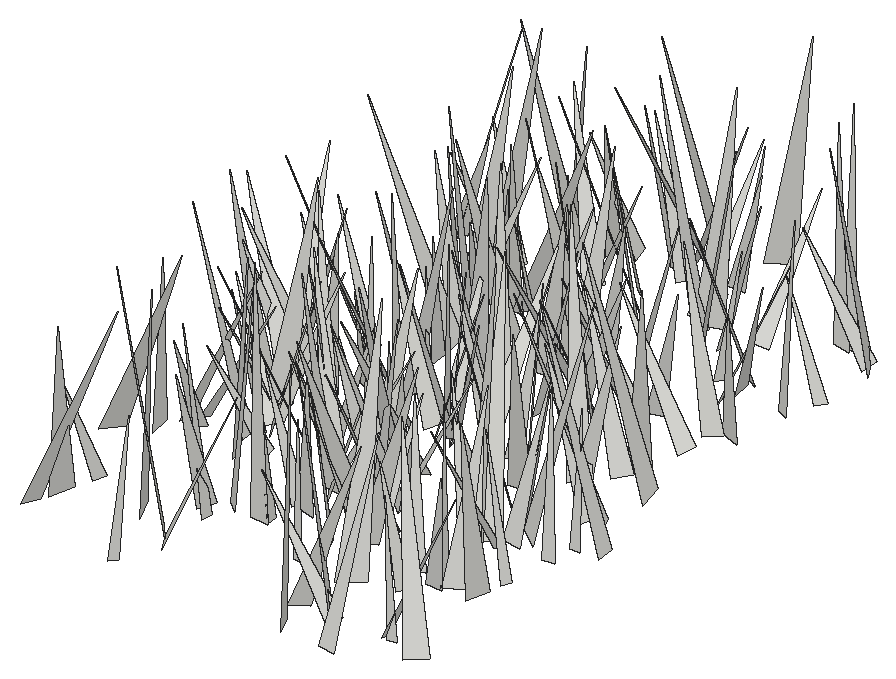
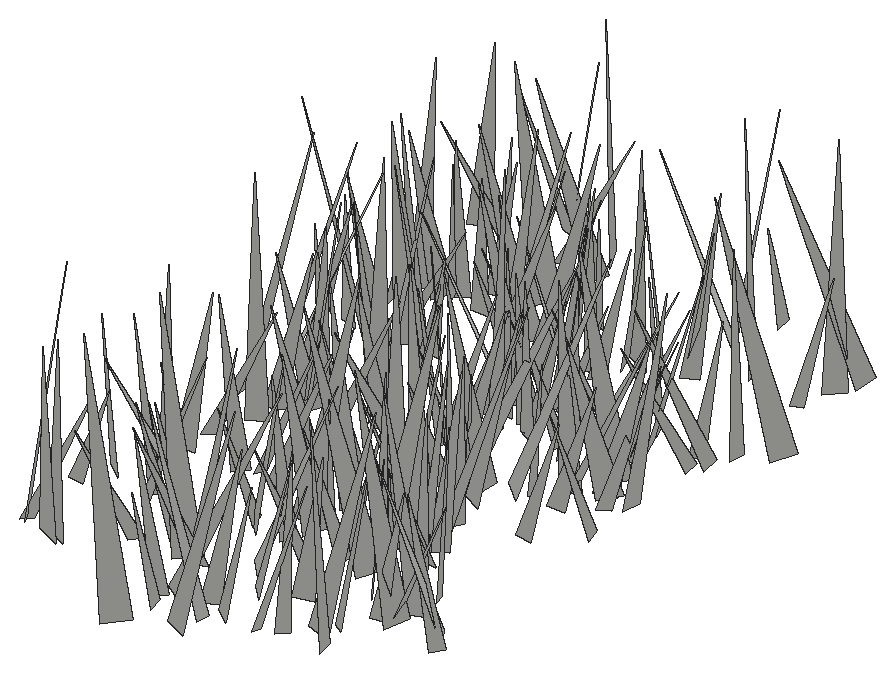
# SketchUp Ruby script. Lengths in inches.
U = 1.inch
M = Sketchup.active_model
def pt(a) = Geom::Point3d.new(a.map { |v| v * U })
def face(e, loops, mat)
  f = e.add_face(loops[0].map { |a| pt(a) })
  loops[1..].each { |l| e.add_face(l.map { |a| pt(a) }).erase! }
  f.material = f.back_material = mat if mat
  f
end
# faces: each face lists its corners as indices into pts; further lists are holes
def faces(e, pts, list, mat = nil) = list.each { |f| face(e, (f[0].is_a?(Array) ? f : [f]).map { |l| l.map { |i| pts[i] } }, mat) }
# xy, xz, yz: faces in a plane at the given z, y or x. An outline is a flat list of corners, or four numbers for a rectangle; further outlines are holes
def ring(l) = l.size == 4 ? [[l[0], l[1]], [l[2], l[1]], [l[2], l[3]], [l[0], l[3]]] : l.each_slice(2).to_a
def flat(e, list, mat, &to3) = list.each { |f| face(e, (f[0].is_a?(Array) ? f : [f]).map { |l| ring(l).map { |u, v| to3.(u, v) } }, mat) }
def xy(e, z, list, mat = nil) = flat(e, list, mat) { |x, y| [x, y, z] }
def xz(e, y, list, mat = nil) = flat(e, list, mat) { |x, z| [x, y, z] }
def yz(e, x, list, mat = nil) = flat(e, list, mat) { |y, z| [x, y, z] }
def lines(e, pts, list) = list.each { |a, b| e.add_line(pt(pts[a]), pt(pts[b])) }
# prism: a flat outline (further loops are holes) pulled along v
def prism(e, loops, v, mat = nil)
  f = face(e, loops, mat); d = Geom::Vector3d.new(v.map { |x| x * U })
  f.pushpull(f.normal.samedirection?(d) ? d.length : -d.length)
end
def box(e, o, s, mat = nil) = prism(e, [[o, [o[0] + s[0], o[1], o[2]], [o[0] + s[0], o[1] + s[1], o[2]], [o[0], o[1] + s[1], o[2]]]], [0, 0, s[2]], mat)
def at(x, y, z, deg = 0) = Geom::Transformation.translation(pt([x, y, z])) * Geom::Transformation.rotation(ORIGIN, Z_AXIS, deg.degrees)
def axes(o, x, y, z) = Geom::Transformation.new([*x, 0, *y, 0, *z, 0, *pt(o).to_a, 1])
def part(name) = M.definitions.add(name)
# library, detail: a bought-in or finely detailed component or shape, given as its bounding box
def library(name, o, s) = part(name).tap { |d| box(d.entities, o, s) }
def detail(e, o, s) = box(e.add_group.entities, o, s)
def put(e, d, t, mat = nil) = e.add_instance(d, t).tap { |i| i.material = mat if mat }
def group(e, t, mat = nil) = e.add_group.tap { |g| g.transformation = t; g.material = mat if mat }.entities
root = M.entities
c1 = part("fur_instance\#9")
p = [[0.8125,0,1.79],[0.67,-0.02,1.48],[0,-0.11,0],[0,0.11,0]]
faces(c1.entities,p,[[0,1,2,3]])
put(root,c1,axes([478.71,327.85,-21.66],[-6.33484,-0.15602,2.15214],[0.09289,6.64883,0.75543],[2.15578,-0.74496,6.29157]))
put(root,c1,axes([477.64,320.11,-21.66],[5.74214,0.07937,1.80023],[0.34922,-5.94743,-0.85168],[-1.76782,-0.91707,5.67918]))
put(root,c1,axes([478.67,313.66,-21.66],[2.63547,-2.52355,0.88422],[-2.24578,-2.7628,-1.19134],[-1.45143,-0.30736,3.44888]))
put(root,c1,axes([477.66,345.35,-21.66],[5.27233,3.79468,0.9806],[3.62511,-5.34626,1.19781],[-1.48988,0.42019,6.38454]))
put(root,c1,axes([480.66,327.67,-21.66],[-3.78677,4.88862,0.77178],[4.90876,3.58599,1.37062],[-0.63111,-1.44081,6.0299]))
put(root,c1,axes([477.02,346.69,-21.66],[2.31724,-3.70248,0.25487],[-3.62607,-2.19471,1.08527],[0.79054,0.78602,4.23086]))
put(root,c1,axes([475.72,318.5,-21.66],[6.5822,-3.48627,0.04021],[-3.46978,-6.5418,0.80411],[0.34104,0.72931,7.40492]))
put(root,c1,axes([479.73,328.98,-21.66],[-4.18916,1.41328,1.44955],[1.84035,4.04661,1.3732],[0.84361,-1.80976,4.20247]))
put(root,c1,axes([478.39,331.58,-21.66],[4.03699,1.00135,1.00845],[0.75439,-4.0837,1.03503],[-1.2044,0.79854,4.02849]))
put(root,c1,axes([477.99,311.26,-21.66],[6.15158,-3.29467,0.71793],[-3.15743,-6.15236,-1.17953],[-1.18361,-0.7112,6.87789]))
put(root,c1,axes([480.25,327.79,-21.66],[-4.33285,5.33033,0.39838],[5.19442,4.31986,-1.30443],[1.26061,0.52067,6.74422]))
put(root,c1,axes([479.34,321.4375,-21.66],[2.09335,-3.21544,0.11512],[-3.16402,-2.08217,-0.6229],[-0.58423,-0.24481,3.78592]))
put(root,c1,axes([481.14,334.13,-21.66],[-1.35537,3.98703,1.26023],[4.07237,0.95801,1.34893],[-0.94888,-1.58348,3.98921]))
put(root,c1,axes([477.34,309.4,-21.66],[6.84085,-1.05323,0.60817],[-1.14548,-6.7472,1.19982],[-0.40871,1.28156,6.81667]))
put(root,c1,axes([481.98,322.28,-21.66],[-6.45817,-1.9042,0.82118],[-2.02073,6.38203,-1.093],[0.4658,1.28531,6.64374]))
put(root,c1,axes([480.9,345.43,-21.66],[-3.67924,-0.76157,0.35539],[-0.68587,3.64327,0.70657],[0.48566,-0.62424,3.6902]))
put(root,c1,axes([478.27,321.625,-21.66],[5.14686,-0.10254,0.48257],[-0.21946,-5.00543,1.27711],[-0.44184,1.29176,4.98695]))
put(root,c1,axes([482.23,328.67,-21.66],[-5.87087,-0.65311,0.1721],[-0.62527,5.82501,0.77566],[0.25536,-0.75237,5.85594]))
put(root,c1,axes([481.77,330.56,-21.66],[-2.38269,3.95567,1.05235],[4.03891,2.07425,1.34786],[-0.66484,-1.57548,4.41677]))
put(root,c1,axes([482.22,324.16,-21.66],[-3.14834,2.92622,0.07201],[2.87738,3.07451,0.86494],[-0.53726,-0.68166,4.21031]))
put(root,c1,axes([478.875,322.49,-21.66],[4.0967,-0.1052,0.02727],[-0.10864,-3.93802,1.12914],[0.00278,1.12946,3.93942]))
put(root,c1,axes([481.6,346,-21.66],[1.42744,-3.53628,2.17287],[-3.81125,-2.02664,-0.79456],[-1.64348,1.62839,3.72982]))
put(root,c1,axes([480.47,342.17,-21.66],[4.23333,1.58778,2.03705],[2.11026,-4.38143,-0.97034],[-1.48911,-1.69519,4.41595]))
put(root,c1,axes([482.51,322.92,-21.66],[-3.84784,-1.19504,0.32807],[-1.23606,3.62421,-1.29571],[-0.08892,1.33363,3.81512]))
put(root,c1,axes([481.8,325.32,-21.66],[-3.17916,-2.57933,0.00353],[-2.53731,3.12837,0.73174],[0.46373,-0.56605,4.02798]))
put(root,c1,axes([480.21,344.3,-21.66],[0.14436,6.2225,2.72909],[6.68972,0.34776,-1.14678],[1.18962,-2.71069,6.11762]))
put(root,c1,axes([480.6,345.7,-21.66],[7.15421,-1.9799,2.12173],[-2.22149,-7.36827,0.61487],[-1.86728,1.18029,7.39761]))
put(root,c1,axes([483.24,349.15,-21.66],[-1.73003,-6.76572,2.01517],[-7.01807,1.42401,-1.24409],[-0.76325,2.2419,6.8717]))
put(root,c1,axes([480.98,326.15,-21.66],[5.12672,-4.5376,2.59386],[-5.0883,-5.16347,1.02416],[-1.19461,2.5199,6.76936]))
put(root,c1,axes([482.89,320.15,-21.66],[-5.05417,-1.27819,2.14403],[-1.86511,5.15169,-1.32541],[1.65892,1.89778,5.04199]))
put(root,c1,axes([484.51,336.86,-21.66],[-7.8071,-1.03462,1.04066],[-0.93299,7.84786,0.80297],[1.13267,-0.66693,7.83431]))
put(root,c1,axes([484.76,323.7,-21.66],[-3.76268,-4.24685,0.11424],[-4.17448,3.66755,-1.15295],[-0.78896,0.84846,5.55555]))
put(root,c1,axes([482.75,347.98,-21.66],[-2.78076,-3.999,1.01738],[-3.97731,2.92434,0.62365],[1.09912,0.46468,4.83071]))
put(root,c1,axes([484.81,330.48,-21.66],[-4.99858,-6.00178,0.67378],[-6.03784,4.94565,-0.739],[-0.1407,0.9901,7.77567]))
put(root,c1,axes([481.91,350.22,-21.66],[6.17707,1.48648,1.9777],[1.80034,-6.34915,-0.85095],[-1.69697,-1.32504,6.29616]))
put(root,c1,axes([482.12,344.14,-21.66],[3.64013,-0.49009,0.65042],[-0.33955,-3.62113,-0.82821],[-0.74023,-0.74902,3.57838]))
put(root,c1,axes([484.16,321.36,-21.66],[-3.93279,-0.23592,0.50656],[-0.05149,3.7386,1.34138],[0.55643,-1.32147,3.70448]))
put(root,c1,axes([483.74,338.1875,-21.66],[3.52477,-3.78027,2.43443],[-3.94318,-4.08529,-0.63451],[-2.1606,1.28874,5.1295]))
put(root,c1,axes([484.87,325.58,-21.66],[-6.05277,2.56522,0.71834],[2.46544,6.06973,-0.90131],[1.00895,0.55714,6.51184]))
put(root,c1,axes([484.54,338.3,-21.66],[-3.5063,-5.04513,2.56803],[-5.65565,3.25438,-1.32851],[0.24851,2.88062,5.99854]))
put(root,c1,axes([482.27,328.67,-21.66],[2.19919,-5.46865,1.19281],[-5.58851,-2.07385,0.79564],[0.31218,1.39943,5.84033]))
put(root,c1,axes([482.7,312.43,-21.66],[6.58164,2.52237,2.667],[2.99732,-6.85363,-0.91486],[-2.11926,-1.85972,6.9888]))
put(root,c1,axes([485.0625,311.23,-21.66],[-5.96506,-5.04673,2.13711],[-5.35643,6.03696,-0.69462],[1.15994,1.92465,7.7826]))
put(root,c1,axes([483.43,344.25,-21.66],[-2.68709,-2.60275,1.28992],[-2.48203,2.97011,0.82256],[1.50922,0.25052,3.6494]))
put(root,c1,axes([482.3,324.28,-21.66],[1.86244,4.7215,0.55373],[4.68693,-1.72429,-1.06173],[0.79484,-0.89561,4.96326]))
put(root,c1,axes([483.55,330.36,-21.66],[-0.85908,-3.57953,0.71794],[-3.54097,0.99653,0.73143],[0.88884,0.51028,3.60778]))
put(root,c1,axes([482.57,323.55,-21.66],[4.81991,2.46867,0.79438],[2.57067,-4.76928,-0.77622],[-0.3421,-1.05666,5.35942]))
put(root,c1,axes([483.27,340.24,-21.66],[4.01305,-1.4697,0.35123],[-1.33059,-3.90931,-1.15533],[-0.71618,-0.97223,4.11458]))
put(root,c1,axes([485.87,313.9,-21.66],[-5.27526,-0.92635,0.94955],[-1.13263,5.17215,-1.24665],[0.69057,1.40673,5.20887]))
put(root,c1,axes([484.89,307.0625,-21.66],[-3.85021,0.78609,0.9669],[0.45373,3.80886,-1.28983],[1.16059,1.11875,3.71193]))
put(root,c1,axes([486.17,346.73,-21.66],[-2.8304,4.89567,0.80261],[4.94903,2.72215,0.8485],[-0.34477,-1.11592,5.59096]))
put(root,c1,axes([485.76,332.74,-21.66],[-2.42816,-5.42807,1.43938],[-5.61543,2.33238,-0.67728],[-0.05217,1.5899,5.90772]))
put(root,c1,axes([483.19,339.5,-21.66],[2.79379,4.96818,0.70977],[4.95175,-2.59669,-1.31495],[0.8165,-1.25148,5.54607]))
put(root,c1,axes([484.66,341.99,-21.66],[-1.17903,-5.46423,1.73554],[-5.62366,1.44698,0.7353],[1.11548,1.51937,5.54141]))
put(root,c1,axes([485.06,314.89,-21.66],[3.85472,-3.45884,0.89823],[-3.26491,-3.94586,-1.18314],[-1.45282,-0.30973,5.04209]))
put(root,c1,axes([486.03,350.9375,-21.66],[-4.24869,-0.73201,1.00331],[-0.4187,4.21079,1.29914],[1.16925,-1.15205,4.11089]))
put(root,c1,axes([484.76,335.1875,-21.66],[4.55576,-0.64185,1.19418],[-0.37344,-4.61891,-1.05794],[-1.3033,-0.92017,4.47746]))
put(root,c1,axes([484.73,350.3,-21.66],[4.79188,-1.27621,1.00499],[-1.01396,-4.79557,-1.25507],[-1.26909,-0.98723,4.79746]))
put(root,c1,axes([486.55,339.17,-21.66],[1.44091,-6.85532,1.40735],[-6.89305,-1.6385,-0.92385],[-1.20912,1.1714,6.94393]))
put(root,c1,axes([486.22,315.65,-21.66],[4.10758,4.73433,2.04961],[4.7509,-4.49256,0.85604],[-2.01089,-0.9434,6.20913]))
put(root,c1,axes([486.87,324,-21.66],[-4.89402,-3.33819,1.83703],[-3.30827,5.20635,0.64726],[1.89038,0.46913,5.88863]))
put(root,c1,axes([488.79,328.04,-21.66],[-3.68425,-5.36529,0.32526],[-5.32374,3.58793,-1.11818],[-0.74155,0.8979,6.41168]))
put(root,c1,axes([485.87,325,-21.66],[3.36091,-1.13304,0.9234],[-1.35023,-3.29337,0.87337],[-0.55977,1.1411,3.43755]))
put(root,c1,axes([487.35,331.08,-21.66],[-3.69275,-0.52533,1.17947],[-0.76187,3.77166,-0.70545],[1.04243,0.89562,3.66261]))
put(root,c1,axes([487.93,322.3125,-21.66],[-0.66847,-3.61729,0.84651],[-3.58891,0.40659,-1.09666],[-0.95975,0.99906,3.51127]))
put(root,c1,axes([488.29,321.97,-21.66],[-2.02202,5.92033,1.45384],[6.05855,1.78151,1.17164],[-0.67672,-1.74024,6.14542]))
put(root,c1,axes([487.82,325.41,-21.66],[1.64216,5.46326,1.64146],[5.44457,-2.0108,1.24565],[-1.70244,-1.16093,5.56707]))
put(root,c1,axes([486.04,331.1,-21.66],[6.43486,-0.85229,1.84553],[-1.08084,-6.62327,0.70985],[-1.72168,0.97247,6.45212]))
put(root,c1,axes([488.4375,350.86,-21.66],[-2.6227,-3.62693,1.52989],[-3.9333,2.34177,-1.19122],[-0.15598,1.93268,4.31442]))
put(root,c1,axes([487.82,325.08,-21.66],[1.8485,-3.49978,1.33816],[-3.45042,-2.17169,-0.91344],[-1.46071,0.70098,3.8511]))
put(root,c1,axes([488.59,347.6875,-21.66],[-3.38469,-3.26483,1.22467],[-3.48648,3.19729,-1.11215],[0.05857,1.65326,4.56929]))
put(root,c1,axes([488.29,315.37,-21.66],[1.87849,6.8023,2.53671],[7.02619,-2.36292,1.13321],[-1.82724,-2.09291,6.96533]))
put(root,c1,axes([488.79,315.82,-21.66],[-4.99068,-1.45127,1.21381],[-1.71677,4.91279,-1.18474],[0.79513,1.49823,5.06058]))
put(root,c1,axes([489.1,329.35,-21.66],[-4.79619,2.23097,0.90337],[2.34699,4.78153,0.65218],[0.53379,-0.97799,5.24932]))
put(root,c1,axes([488.96,338.85,-21.66],[0.98464,3.25356,1.70885],[3.23357,-1.6077,1.19779],[-1.74639,-1.14237,3.18127]))
put(root,c1,axes([490.18,345.78,-21.66],[-4.77204,-4.71706,0.72174],[-4.75307,4.60775,-1.31181],[-0.42413,1.43592,6.58044]))
put(root,c1,axes([485.13,342.29,-21.66],[6.73019,-3.63445,0.24466],[-3.63894,-6.68481,0.79754],[0.16506,0.81773,7.60715]))
put(root,c1,axes([488.13,332.15,-21.66],[-2.89622,3.26829,0.45856],[3.08153,2.89643,-1.18106],[1.18158,0.4572,4.20415]))
put(root,c1,axes([486.59,336.1,-21.66],[1.17018,-6.95871,1.51726],[-7.0392,-0.89595,1.31981],[1.08411,1.69372,6.93189]))
put(root,c1,axes([485.75,310.34,-21.66],[5.05169,2.87341,0.23488],[2.86098,-4.93803,-1.1233],[0.35552,-1.09113,5.70213]))
put(root,c1,axes([488.9,318.11,-21.66],[-2.91756,2.69263,1.56889],[3.08399,2.80363,0.92331],[0.448,-1.76443,3.86133]))
put(root,c1,axes([487.09,342.07,-21.66],[3.48145,-1.92251,0.90917],[-2.10367,-3.36896,0.93158],[-0.31179,1.26381,3.86636]))
put(root,c1,axes([489.62,353.47,-21.66],[-2.51805,-6.35566,1.6356],[-6.55451,2.34778,-0.96776],[-0.32873,1.87181,6.76746]))
put(root,c1,axes([488.78,334.05,-21.66],[-4.40075,-1.21691,1.44212],[-0.98766,4.60363,0.87078],[1.60783,-0.50284,4.4821]))
put(root,c1,axes([489.28,320.42,-21.66],[1.25077,5.74635,3.18749],[6.40163,-1.79789,0.7292],[-1.48314,-2.91412,5.83551]))
put(root,c1,axes([487.72,344.14,-21.66],[4.13014,0.16234,0.60229],[0.00137,-4.03539,1.07832],[-0.62379,1.06603,3.99019]))
put(root,c1,axes([489.79,350.22,-21.66],[-3.61147,3.35043,1.62323],[3.67501,3.56996,0.80783],[0.59541,-1.71259,4.85958]))
put(root,c1,axes([489.76,339.82,-21.66],[1.9045,4.44389,1.45881],[4.34306,-2.26488,1.22946],[-1.73613,-0.79091,4.67587]))
put(root,c1,axes([490.03,329.28,-21.66],[-4.76219,-1.42096,1.84075],[-1.91994,4.76946,-1.2853],[1.31199,1.82182,4.80058]))
put(root,c1,axes([490.82,328.77,-21.66],[-2.4507,-4.58404,1.24543],[-4.71435,2.17524,-1.27033],[-0.58261,1.68089,5.0404]))
put(root,c1,axes([491.95,350.61,-21.66],[-3.14306,-6.22127,0.26286],[-6.12359,3.03481,-1.39417],[-1.12913,0.859,6.8293]))
put(root,c1,axes([490.36,324.92,-21.66],[-3.60643,-6.53276,3.39182],[-7.2869,3.70246,-0.61691],[1.0404,3.28673,7.43658]))
put(root,c1,axes([490.78,333.09,-21.66],[-0.82841,6.75025,1.93378],[7.00258,0.65031,0.72978],[-0.51887,-2.00072,6.76162]))
put(root,c1,axes([488.95,324.23,-21.66],[1.24719,-3.91493,0.4967],[-3.8954,-1.13791,0.81231],[0.63182,0.71228,4.02769]))
put(root,c1,axes([489.92,328.53,-21.66],[3.50829,2.33455,0.59392],[2.17247,-3.51961,1.00185],[-1.04078,0.52272,4.09323]))
put(root,c1,axes([490.28,340.63,-21.66],[-4.55508,3.55475,2.05706],[3.40532,4.98624,-1.07596],[2.29598,-0.34303,5.67691]))
put(root,c1,axes([489.66,317.6,-21.66],[-0.19463,-4.95849,1.24268],[-5.00803,0.4343,0.94858],[1.02496,1.18047,4.8708]))
put(root,c1,axes([488.2,322.82,-21.66],[4.34126,2.62004,0.01209],[2.52851,-4.18338,-1.34808],[0.68659,-1.1602,4.88813]))
put(root,c1,axes([490.1875,324.2,-21.66],[-1.33091,-4.34516,1.37723],[-4.35803,1.6335,0.94222],[1.33595,0.99989,4.44566]))
put(root,c1,axes([491.89,318.91,-21.66],[-4.72142,-2.258,0.83052],[-2.14472,4.77905,0.80066],[1.09019,-0.37724,5.17198]))
put(root,c1,axes([491.8125,324.75,-21.66],[0.91658,-6.09487,0.23316],[-5.96683,-0.94489,-1.24341],[-1.26442,0.04079,6.03668]))
put(root,c1,axes([491.44,339.9,-21.66],[2.47706,-6.70826,1.39737],[-6.69174,-2.68793,-1.04158],[-1.47445,0.92925,7.07472]))
put(root,c1,axes([489.58,319.64,-21.66],[4.36053,2.62617,0.62372],[2.69593,-4.29581,-0.7602],[-0.13318,-0.97427,5.03319]))
put(root,c1,axes([490.16,322.64,-21.66],[-1.02594,6.32348,2.52203],[6.58274,1.57191,-1.26344],[1.73626,-2.22313,6.28034]))
put(root,c1,axes([491.9375,330.51,-21.66],[1.8151,-3.86013,1.55176],[-3.9232,-2.15155,-0.76319],[-1.38458,1.03602,4.19675]))
put(root,c1,axes([489.07,351.78,-21.66],[6.07626,0.90493,0.17774],[0.92213,-5.94508,-1.25588],[0.01299,-1.26833,6.01354]))
put(root,c1,axes([490.71,328.75,-21.66],[4.61711,2.95667,1.94744],[3.35791,-4.67134,-0.86895],[-1.12198,-1.8135,5.41336]))
put(root,c1,axes([492.01,319.22,-21.66],[1.78326,-6.33726,0.7797],[-6.26284,-1.89367,-1.06754],[-1.24322,0.44943,6.49625]))
put(root,c1,axes([490.27,337.44,-21.66],[2.54415,-5.74451,1.38415],[-5.89364,-2.3587,1.04378],[0.42454,1.68081,6.19537]))
put(root,c1,axes([490.88,323.97,-21.66],[-1.24529,-7.71146,0.7872],[-7.61167,1.36728,1.35282],[1.46589,0.54863,7.69333]))
put(root,c1,axes([492.83,315.96,-21.66],[-3.64875,-2.02244,1.121],[-2.25149,3.58457,-0.86132],[0.52696,1.3118,4.08188]))
put(root,c1,axes([491.42,331.5,-21.66],[-1.51981,5.35977,0.02073],[5.22969,1.48762,-1.21441],[1.17387,0.31183,5.43711]))
put(root,c1,axes([490.78,342.24,-21.66],[2.11868,-4.0714,0.72457],[-4.11944,-2.00647,0.77101],[0.3627,0.99394,4.52445]))
put(root,c1,axes([490.96,322.25,-21.66],[-2.2184,-4.85625,2.50772],[-5.03427,2.86928,1.10295],[2.1279,1.72546,5.22379]))
put(root,c1,axes([492.61,313.25,-21.66],[1.15906,3.62365,1.13013],[3.60388,-1.42153,0.86183],[-1.19166,-0.77453,3.7056]))
put(root,c1,axes([493.1,342.26,-21.66],[-3.89447,-3.70378,1.65585],[-4.00703,3.87088,-0.766],[0.63525,1.71028,5.3196]))
put(root,c1,axes([492.05,352.12,-21.66],[3.63401,0.67625,1.41653],[0.37628,-3.84346,0.86953],[-1.5239,0.6636,3.59267]))
put(root,c1,axes([493.05,321.54,-21.66],[-5.52274,-3.05851,1.02558],[-2.84433,5.57616,1.31266],[1.52186,-0.67738,6.17511]))
put(root,c1,axes([490.95,328.95,-21.66],[4.30698,0.82715,0.77594],[0.97071,-4.26434,-0.84231],[-0.5865,-0.98365,4.30404]))
put(root,c1,axes([494.1,346.12,-21.66],[-7.25051,-1.24633,1.39987],[-1.43303,7.2913,-0.93068],[1.20805,1.16894,7.29774]))
put(root,c1,axes([494.2,336.17,-21.66],[-1.56968,-5.60909,0.11931],[-5.50885,1.51747,-1.1357],[-1.06238,0.41882,5.71278]))
put(root,c1,axes([492.67,333.83,-21.66],[4.75143,0.92242,1.33841],[0.70934,-4.89704,0.85681],[-1.46255,0.62163,4.7637]))
put(root,c1,axes([492.85,347.27,-21.66],[-0.26942,5.43204,0.24352],[5.36362,0.30555,-0.88154],[0.89325,-0.19629,5.36679]))
put(root,c1,axes([493.05,320.1,-21.66],[-0.85161,3.55792,0.87868],[3.50079,1.05663,-0.88551],[1.08413,-0.61714,3.54963]))
put(root,c1,axes([492.45,351.21,-21.66],[1.94389,-4.04886,0.80465],[-4.08173,-1.75236,1.04312],[0.61659,1.16421,4.36851]))
put(root,c1,axes([493.51,341.58,-21.66],[3.85077,0.95797,1.10657],[0.6489,-3.90916,1.12606],[-1.31192,0.87829,3.80501]))
put(root,c1,axes([494.09,319.68,-21.66],[-2.87377,-5.9267,0.11201],[-5.79461,2.83495,1.33509],[1.24935,-0.48389,6.44995]))
put(root,c1,axes([492.52,354.9,-21.66],[5.49312,-5.94068,1.74056],[-6.16398,-5.4638,0.80479],[-0.57141,1.8305,8.05098]))
put(root,c1,axes([495.29,337.94,-21.66],[-1.01525,-4.25558,0.24661],[-4.20456,0.95799,-0.77812],[-0.70176,0.41691,4.30525]))
put(root,c1,axes([494.67,335.9,-21.66],[-2.5051,-3.46967,0.23869],[-3.39401,2.50314,0.76559],[0.75915,-0.25846,4.21047]))
put(root,c1,axes([493.87,347.07,-21.66],[-3.12669,6.25889,3.83958],[6.87271,3.96367,-0.86451],[2.58493,-2.9678,6.9428]))
put(root,c1,axes([494.65,329.27,-21.66],[3.28542,-2.52777,1.83261],[-2.97263,-3.34603,0.71392],[-0.95477,1.71946,4.08337]))
put(root,c1,axes([496.68,337.32,-21.66],[-4.54566,0.43172,0.55069],[0.54174,4.46219,0.97364],[0.44289,-1.02717,4.4611]))
put(root,c1,axes([495.05,344.9,-21.66],[4.98467,2.72403,1.68688],[2.57744,-5.26236,0.88159],[-1.90334,0.00786,5.61161]))
put(root,c1,axes([493.16,321.33,-21.66],[4.26257,2.91433,0.00484],[2.86478,-4.18851,-0.95515],[0.53516,-0.79116,5.0745]))
put(root,c1,axes([496.79,333.6,-21.66],[-6.4254,-4.61842,2.37343],[-5.01235,6.50279,-0.91585],[1.35622,2.15235,7.85982]))
put(root,c1,axes([493.86,335.9,-21.66],[3.98681,-3.04122,0.56389],[-3.08769,-3.85909,1.01744],[0.18196,1.14894,4.91004]))
put(root,c1,axes([496.16,324.85,-21.66],[-3.36385,-0.86607,1.07357],[-0.51946,3.41676,1.12873],[1.27781,-0.89095,3.28504]))
put(root,c1,axes([494.32,316.99,-21.66],[4.99795,-3.82327,1.26682],[-4.01963,-4.86241,1.18375],[-0.25457,1.71502,6.18026]))
put(root,c1,axes([496.3,313.23,-21.66],[5.95771,-4.00613,4.25574],[-5.13988,-6.48421,1.09155],[-2.78246,3.40011,7.09591]))
put(root,c1,axes([497.56,321.49,-21.66],[-1.2405,4.10694,0.41743],[4.03089,1.11105,1.04764],[-0.89058,-0.69186,4.16031]))
put(root,c1,axes([496.49,307.25,-21.66],[6.19858,3.66698,3.16063],[3.75526,-6.8827,0.6206],[-3.05522,-1.01998,7.17523]))
put(root,c1,axes([498.41,309.24,-21.66],[-4.58076,1.47717,0.18742],[1.47131,4.39705,1.30451],[-0.22897,-1.29786,4.63288]))
put(root,c1,axes([497.93,309.54,-21.66],[-5.99226,-3.56649,1.99916],[-3.93709,5.99,-1.11487],[1.10264,2.00593,6.88361]))
put(root,c1,axes([495.93,345.62,-21.66],[4.26152,0.65659,1.09682],[0.47447,-4.35714,0.76482],[-1.18701,0.6156,4.24343]))
put(root,c1,axes([495.87,328.95,-21.66],[4.89735,3.35239,2.18214],[3.80193,-4.97328,-0.89225],[-1.24321,-2.00306,5.86741]))
put(root,c1,axes([499.02,329.51,-21.66],[-7.08431,2.74004,0.68893],[2.60293,7.0529,-1.28499],[1.09872,0.95845,7.48626]))
put(root,c1,axes([497.29,322.35,-21.66],[-5.34624,-2.21651,3.3319],[-3.00843,5.89263,-0.90721],[2.6389,2.22728,5.71596]))
put(root,c1,axes([498.36,316.29,-21.66],[-0.93822,4.8343,1.08723],[4.93478,0.81164,0.64956],[-0.44769,-1.18472,4.88147]))
put(root,c1,axes([495.74,309.47,-21.66],[5.04993,-3.13211,0.88061],[-3.25342,-4.87587,1.31476],[-0.02926,1.58216,5.79512]))
put(root,c1,axes([497.95,324.98,-21.66],[-3.94207,-4.94022,1.13908],[-4.81769,4.09962,1.10733],[1.57897,0.1748,6.2225]))
put(root,c1,axes([497.36,347.12,-21.66],[-1.55041,4.4226,0.08121],[4.26043,1.51619,-1.23272],[1.18941,0.33394,4.52145]))
put(root,c1,axes([499.59,343.64,-21.66],[-3.22494,-3.97651,0.65226],[-4.0077,3.07801,-1.05003],[-0.42001,1.16258,5.01102]))
put(root,c1,axes([497.95,342.8,-21.66],[-3.37958,0.77927,1.41196],[0.41341,3.58754,-0.99047],[1.55884,0.73803,3.32382]))
put(root,c1,axes([498.42,321.29,-21.66],[2.96295,7.07925,2.39249],[7.30087,-3.29107,0.69644],[-1.59283,-1.91622,7.64263]))
put(root,c1,axes([497.01,326.88,-21.66],[1.92624,-6.27783,0.49509],[-6.26935,-1.863,0.76884],[0.59288,0.69623,6.52153]))
put(root,c1,axes([499.21,321.24,-21.66],[-5.51425,5.90533,1.65371],[5.90522,5.71303,-0.71018],[1.6541,-0.70927,8.04832]))
put(root,c1,axes([500.17,321.06,-21.66],[-1.30366,-3.70433,0.26528],[-3.50778,1.13584,-1.37745],[-1.21983,0.69265,3.67753]))
put(root,c1,axes([499.08,314.3,-21.66],[2.35364,-2.97334,1.61897],[-3.0072,-2.74184,-0.66374],[-1.55518,0.80187,3.73361]))
put(root,c1,axes([500.51,331.3,-21.66],[-3.89894,3.87426,1.21258],[4.05705,3.77806,0.97396],[0.14352,-1.54866,5.40953]))
put(root,c1,axes([497.64,337.78,-21.66],[2.67886,-4.09104,0.57639],[-4.11516,-2.58128,0.80469],[0.36641,0.91951,4.82342]))
put(root,c1,axes([501.49,335.66,-21.66],[-4.58774,2.19144,0.09862],[2.15217,4.45217,1.18567],[-0.42461,-1.11142,4.94408]))
put(root,c1,axes([498.74,330.14,-21.66],[4.04203,-2.33275,1.48439],[-2.65208,-4.01454,0.91276],[-0.78205,1.55722,4.57675]))
put(root,c1,axes([500.52,316.03,-21.66],[-4.80095,-0.85986,1.55653],[-1.24807,4.82151,-1.18603],[1.26668,1.49164,4.73094]))
put(root,c1,axes([499.92,306.59,-21.66],[1.80185,5.93958,0.37976],[5.89361,-1.83593,0.75111],[-0.82954,-0.14229,6.16126]))
put(root,c1,axes([501.54,337.82,-21.66],[-2.10663,5.00928,1.58804],[5.23429,1.84857,1.1125],[-0.46582,-1.88217,5.31913]))
put(root,c1,axes([500.87,349.69,-21.66],[1.52535,6.05061,2.3847],[6.37233,-1.8801,0.69429],[-1.30004,-2.1163,6.20117]))
put(root,c1,axes([503.08,326.66,-21.66],[-6.30191,-3.29477,0.26908],[-3.30318,6.25333,-0.79169],[-0.13009,0.82599,7.06702]))
put(root,c1,axes([501.28,349.83,-21.66],[1.52535,6.57132,1.88983],[6.63248,-1.89273,1.22809],[-1.66251,-1.52175,6.63331]))
put(root,c1,axes([499.5,340.87,-21.66],[4.18382,1.92252,0.07247],[1.86113,-4.08842,1.01327],[-0.48737,0.89131,4.49152]))
put(root,c1,axes([502.11,326.51,-21.66],[-4.9541,1.83691,1.27432],[2.05779,4.95762,0.85363],[0.87385,-1.26054,5.21428]))
put(root,c1,axes([500.17,315.54,-21.66],[0.87128,-4.23502,0.75689],[-4.24446,-0.72019,0.85631],[0.702,0.90186,4.23807]))
put(root,c1,axes([501.09,316.1,-21.66],[-4.2045,3.84796,1.64776],[3.68267,4.51063,-1.13666],[1.98995,-0.21727,5.58504]))
put(root,c1,axes([502.08,309.53,-21.66],[0.5553,3.90242,1.15183],[3.90207,-0.84018,0.96535],[-1.15302,-0.96393,3.8217]))
put(root,c1,axes([500,323.38,-21.66],[5.07227,1.20948,1.05659],[1.39553,-5.05165,-0.91676],[-0.7948,-1.15114,5.13326]))
put(root,c1,axes([500.46,321.82,-21.66],[0.08637,4.97569,1.67082],[5.15736,0.22998,-0.95146],[0.97504,-1.65717,4.88463]))
put(root,c1,axes([499.62,342.69,-21.66],[4.97063,-0.22915,0.23226],[-0.15729,-4.7897,-1.3593],[-0.28585,-1.34904,4.78665]))
put(root,c1,axes([502.98,318.27,-21.66],[-4.26519,0.30143,0.24037],[0.24291,4.17451,-0.92459],[0.29939,0.9072,4.17466]))
put(root,c1,axes([503.07,330.52,-21.66],[-7.82049,-1.65264,1.82204],[-1.48703,8.01344,0.88582],[1.95953,-0.51451,7.94397]))
put(root,c1,axes([503.34,349.01,-21.66],[-4.40105,0.97982,0.44244],[1.06612,4.21791,1.26401],[0.13855,-1.33202,4.328]))
put(root,c1,axes([500.36,332.98,-21.66],[1.17808,-6.7396,1.1437],[-6.76699,-0.98532,1.16408],[0.96855,1.31342,6.74203]))
put(root,c1,axes([500.69,322.99,-21.66],[4.61104,6.12434,1.67223],[6.3457,-4.50796,-0.9879],[-0.18966,-1.93296,7.60219]))
put(root,c1,axes([503.1875,321.59,-21.66],[0.59003,4.76484,1.13067],[4.77949,-0.80843,0.91275],[-1.06703,-0.9864,4.71367]))
put(root,c1,axes([503.9,344.14,-21.66],[-1.40668,3.30295,0.84871],[3.29754,1.08331,1.24951],[-0.86952,-1.23511,3.36556]))
put(root,c1,axes([502.96,342.02,-21.66],[2.73063,4.59292,1.67983],[4.59916,-3.06583,0.90635],[-1.66266,-0.93747,5.2659]))
put(root,c1,axes([505.15,324.07,-21.66],[-7.20158,-1.52489,0.67202],[-1.60184,7.15641,-0.92717],[0.45935,1.04894,7.30263]))
put(root,c1,axes([501.49,309.75,-21.66],[4.45385,0.90104,0.34779],[0.77968,-4.32278,1.21461],[-0.57002,1.12752,4.37874]))
put(root,c1,axes([504.36,308.78,-21.66],[-3.46559,5.8146,1.30946],[5.95968,3.40104,0.67057],[0.08042,-1.46897,6.73574]))
put(root,c1,axes([503.59,323.37,-21.66],[0.89714,3.83975,1.01573],[3.88067,-1.06922,0.61438],[-0.84607,-0.83267,3.89501]))
put(root,c1,axes([503.45,348.89,-21.66],[-6.01698,-4.0059,2.23214],[-3.85326,6.41302,1.12219],[2.48637,0.24439,7.14087]))
put(root,c1,axes([502.62,316.26,-21.66],[5.63565,-3.00774,1.4531],[-2.80235,-5.80815,-1.15361],[-1.81792,-0.37081,6.28301]))
put(root,c1,axes([502.48,338.12,-21.66],[-0.50328,-4.91347,1.0032],[-4.85841,0.72759,1.12622],[1.24277,0.85458,4.80907]))
